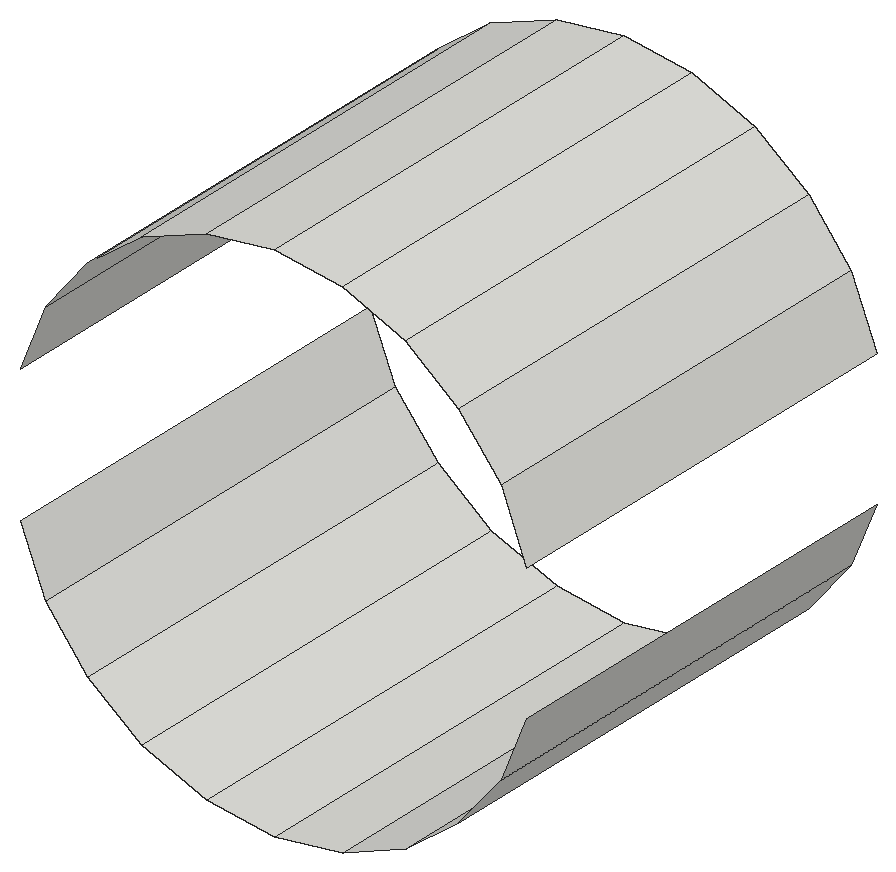
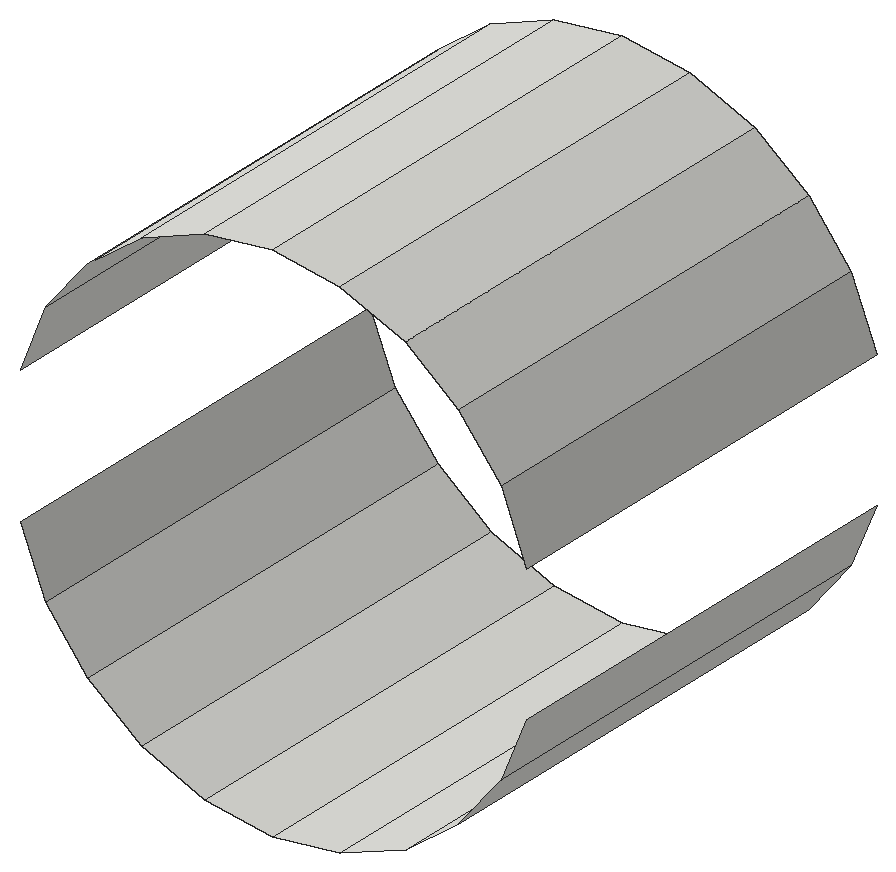
# SketchUp Ruby script. Lengths in inches.
U = 1.inch
M = Sketchup.active_model
def pt(a) = Geom::Point3d.new(a.map { |v| v * U })
def face(e, loops, mat)
  f = e.add_face(loops[0].map { |a| pt(a) })
  loops[1..].each { |l| e.add_face(l.map { |a| pt(a) }).erase! }
  f.material = f.back_material = mat if mat
  f
end
# faces: each face lists its corners as indices into pts; further lists are holes
def faces(e, pts, list, mat = nil) = list.each { |f| face(e, (f[0].is_a?(Array) ? f : [f]).map { |l| l.map { |i| pts[i] } }, mat) }
# xy, xz, yz: faces in a plane at the given z, y or x. An outline is a flat list of corners, or four numbers for a rectangle; further outlines are holes
def ring(l) = l.size == 4 ? [[l[0], l[1]], [l[2], l[1]], [l[2], l[3]], [l[0], l[3]]] : l.each_slice(2).to_a
def flat(e, list, mat, &to3) = list.each { |f| face(e, (f[0].is_a?(Array) ? f : [f]).map { |l| ring(l).map { |u, v| to3.(u, v) } }, mat) }
def xy(e, z, list, mat = nil) = flat(e, list, mat) { |x, y| [x, y, z] }
def xz(e, y, list, mat = nil) = flat(e, list, mat) { |x, z| [x, y, z] }
def yz(e, x, list, mat = nil) = flat(e, list, mat) { |y, z| [x, y, z] }
def lines(e, pts, list) = list.each { |a, b| e.add_line(pt(pts[a]), pt(pts[b])) }
# prism: a flat outline (further loops are holes) pulled along v
def prism(e, loops, v, mat = nil)
  f = face(e, loops, mat); d = Geom::Vector3d.new(v.map { |x| x * U })
  f.pushpull(f.normal.samedirection?(d) ? d.length : -d.length)
end
def box(e, o, s, mat = nil) = prism(e, [[o, [o[0] + s[0], o[1], o[2]], [o[0] + s[0], o[1] + s[1], o[2]], [o[0], o[1] + s[1], o[2]]]], [0, 0, s[2]], mat)
def at(x, y, z, deg = 0) = Geom::Transformation.translation(pt([x, y, z])) * Geom::Transformation.rotation(ORIGIN, Z_AXIS, deg.degrees)
def axes(o, x, y, z) = Geom::Transformation.new([*x, 0, *y, 0, *z, 0, *pt(o).to_a, 1])
def part(name) = M.definitions.add(name)
# library, detail: a bought-in or finely detailed component or shape, given as its bounding box
def library(name, o, s) = part(name).tap { |d| box(d.entities, o, s) }
def detail(e, o, s) = box(e.add_group.entities, o, s)
def put(e, d, t, mat = nil) = e.add_instance(d, t).tap { |i| i.material = mat if mat }
def group(e, t, mat = nil) = e.add_group.tap { |g| g.transformation = t; g.material = mat if mat }.entities
root = M.entities
p = [[2611.93,801.78,132.03],[2612.21,801.78,131.92],[2612.21,799.91,131.92],[2611.93,799.91,132.03],[2612.5,801.78,131.88],[2612.5,799.91,131.88],
  [2612.79,801.78,131.92],[2612.79,799.91,131.92],[2613.06,801.78,132.03],[2613.06,799.91,132.03],[2611.7,801.78,132.21],[2611.7,799.91,132.21],
  [2613.29,801.78,132.21],[2613.29,799.91,132.21],[2611.52,801.78,132.44],[2611.52,799.91,132.44],[2613.47,801.78,132.44],[2613.47,799.91,132.44],
  [2611.41,801.78,132.71],[2611.41,799.91,132.71],[2613.58,801.78,132.71],[2613.58,799.91,132.71],[2611.52,801.78,133.57],[2611.41,801.78,133.29],
  [2611.41,799.91,133.29],[2611.52,799.91,133.57],[2613.58,801.78,133.29],[2613.47,801.78,133.57],[2613.47,799.91,133.57],[2613.58,799.91,133.29],
  [2611.7,801.78,133.8],[2611.7,799.91,133.8],[2613.29,801.78,133.8],[2613.29,799.91,133.8],[2611.93,801.78,133.98],[2611.93,799.91,133.98],
  [2613.06,801.78,133.98],[2613.06,799.91,133.98],[2612.21,801.78,134.09],[2612.21,799.91,134.09],[2612.79,801.78,134.09],[2612.79,799.91,134.09],
  [2612.5,801.78,134.13],[2612.5,799.91,134.13]]
faces(root,p,[[0,1,2,3],[1,4,5,2],[4,6,7,5],[6,8,9,7],[10,0,3,11],[8,12,13,9],[14,10,11,15],[12,16,17,13],
  [18,14,15,19],[16,20,21,17],[22,23,24,25],[26,27,28,29],[30,22,25,31],[27,32,33,28],[34,30,31,35],[32,36,37,33],
  [38,34,35,39],[36,40,41,37],[42,38,39,43],[40,42,43,41]])
